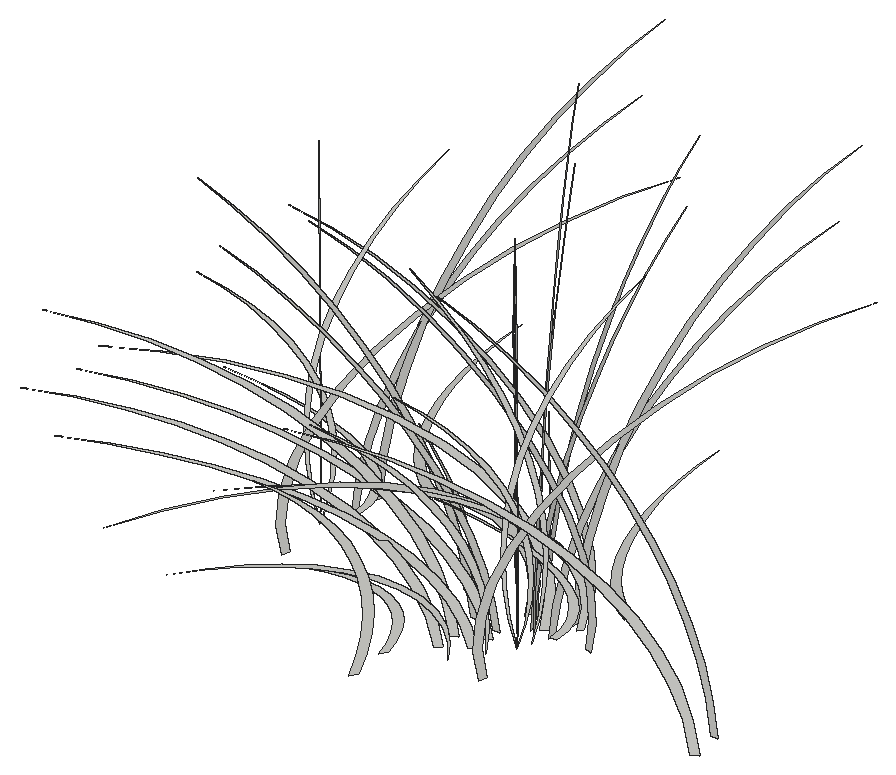
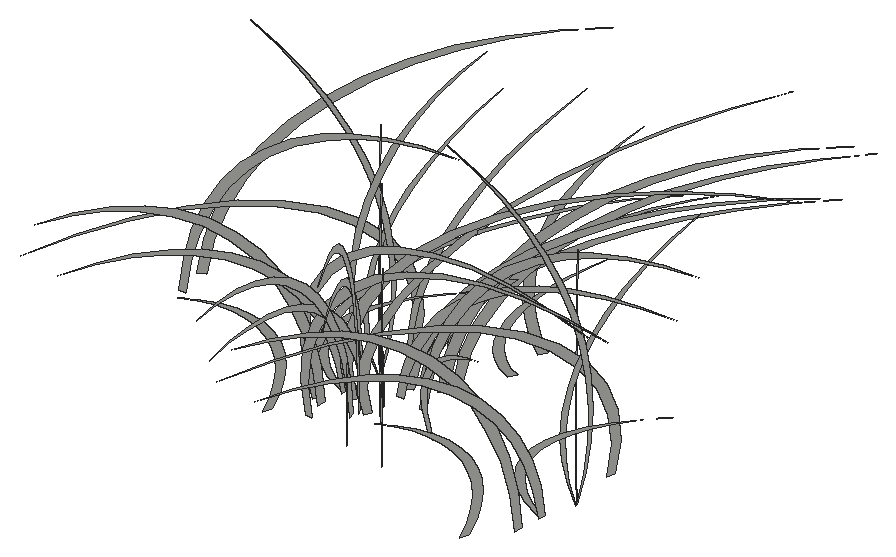
# SketchUp Ruby script. Lengths in inches.
U = 1.inch
M = Sketchup.active_model
def pt(a) = Geom::Point3d.new(a.map { |v| v * U })
def face(e, loops, mat)
  f = e.add_face(loops[0].map { |a| pt(a) })
  loops[1..].each { |l| e.add_face(l.map { |a| pt(a) }).erase! }
  f.material = f.back_material = mat if mat
  f
end
# faces: each face lists its corners as indices into pts; further lists are holes
def faces(e, pts, list, mat = nil) = list.each { |f| face(e, (f[0].is_a?(Array) ? f : [f]).map { |l| l.map { |i| pts[i] } }, mat) }
# xy, xz, yz: faces in a plane at the given z, y or x. An outline is a flat list of corners, or four numbers for a rectangle; further outlines are holes
def ring(l) = l.size == 4 ? [[l[0], l[1]], [l[2], l[1]], [l[2], l[3]], [l[0], l[3]]] : l.each_slice(2).to_a
def flat(e, list, mat, &to3) = list.each { |f| face(e, (f[0].is_a?(Array) ? f : [f]).map { |l| ring(l).map { |u, v| to3.(u, v) } }, mat) }
def xy(e, z, list, mat = nil) = flat(e, list, mat) { |x, y| [x, y, z] }
def xz(e, y, list, mat = nil) = flat(e, list, mat) { |x, z| [x, y, z] }
def yz(e, x, list, mat = nil) = flat(e, list, mat) { |y, z| [x, y, z] }
def lines(e, pts, list) = list.each { |a, b| e.add_line(pt(pts[a]), pt(pts[b])) }
# prism: a flat outline (further loops are holes) pulled along v
def prism(e, loops, v, mat = nil)
  f = face(e, loops, mat); d = Geom::Vector3d.new(v.map { |x| x * U })
  f.pushpull(f.normal.samedirection?(d) ? d.length : -d.length)
end
def box(e, o, s, mat = nil) = prism(e, [[o, [o[0] + s[0], o[1], o[2]], [o[0] + s[0], o[1] + s[1], o[2]], [o[0], o[1] + s[1], o[2]]]], [0, 0, s[2]], mat)
def at(x, y, z, deg = 0) = Geom::Transformation.translation(pt([x, y, z])) * Geom::Transformation.rotation(ORIGIN, Z_AXIS, deg.degrees)
def axes(o, x, y, z) = Geom::Transformation.new([*x, 0, *y, 0, *z, 0, *pt(o).to_a, 1])
def part(name) = M.definitions.add(name)
# library, detail: a bought-in or finely detailed component or shape, given as its bounding box
def library(name, o, s) = part(name).tap { |d| box(d.entities, o, s) }
def detail(e, o, s) = box(e.add_group.entities, o, s)
def put(e, d, t, mat = nil) = e.add_instance(d, t).tap { |i| i.material = mat if mat }
def group(e, t, mat = nil) = e.add_group.tap { |g| g.transformation = t; g.material = mat if mat }.entities
root = M.entities
g1 = group(root,at(405.82,272.46,0))
p = [[-9.01,-2.98,7.88],[-7.3,-2.41,7.38],[-5.75,-1.9,6.83],[-4.38,-1.45,6.24],[-3.2,-1.06,5.62],[-2.23,-0.74,4.96],
  [-1.47,-0.49,4.27],[-0.92,-0.31,3.57],[-0.61,-0.2,2.86],[-0.51,-0.17,2.13],[-0.65,-0.21,1.41],[-1.01,-0.33,0.7],
  [-1.6,-0.53,0],[-1.21,-0.4,0],[-0.54,-0.18,0.69],[-0.12,-0.04,1.4],[0.06,0.02,2.13],[-0.02,-0.01,2.85],
  [-0.35,-0.11,3.58],[-0.92,-0.3,4.29],[-1.73,-0.57,4.98],[-2.78,-0.92,5.64],[-4.05,-1.34,6.27],[-5.52,-1.82,6.86],
  [-7.18,-2.375,7.4]]
faces(g1,p,[[0,1,2,3,4,5,6,7,8,9,10,11,12,13,14,15,16,17,18,19,20,21,22,23,24]])
g2 = group(root,at(404.15,269.07,0))
p = [[-0.6,0.73,0],[-0.27,0.33,1.77],[-0.07,0.08,3.57],[0,0,5.36],[-0.07,0.08,7.16],[-0.27,0.32,8.95],
  [-0.6,0.73,10.73],[-1.06,1.29,12.48],[-1.65,2.01,14.2],[-2.37,2.88,15.88],[-3.21,3.91,17.52],[-4.17,5.08,19.1],
  [-5.25,6.39,20.625],[-4.23,5.15,19.08],[-3.33,4.05,17.48],[-2.53,3.08,15.83],[-1.84,2.25,14.15],[-1.27,1.55,12.43],
  [-0.82,1,10.6875],[-0.48,0.59,8.92],[-0.27,0.32,7.14],[-0.17,0.21,5.35],[-0.19,0.24,3.5625],[-0.34,0.41,1.78]]
faces(g2,p,[[0,1,2,3,4,5,6,7,8,9,10,11,12,13,14,15,16,17,18,19,20,21,22,23]])
g3 = group(root,at(404.07,270.6,0))
p = [[-0.52,-0.79,0],[-0.23,-0.35,1.51],[-0.06,-0.09,3.03],[0,0,4.56],[-0.06,-0.09,6.09],[-0.23,-0.35,7.61],
  [-0.52,-0.79,9.12],[-0.92,-1.39,10.61],[-1.43,-2.17,12.07],[-2.05,-3.12,13.5],[-2.78,-4.23,14.89],[-3.61,-5.49,16.24],
  [-4.54,-6.91,17.53],[-3.66,-5.57,16.21],[-2.88,-4.38,14.86],[-2.1875,-3.33,13.46],[-1.6,-2.43,12.03],[-1.1,-1.68,10.57],
  [-0.71,-1.08,9.08],[-0.42,-0.64,7.58],[-0.23,-0.35,6.07],[-0.15,-0.22,4.55],[-0.17,-0.25,3.03],[-0.29,-0.44,1.51]]
faces(g3,p,[[0,1,2,3,4,5,6,7,8,9,10,11,12,13,14,15,16,17,18,19,20,21,22,23]])
g4 = group(root,at(404.18,271.82,0))
p = [[1.63,20.71,16.73],[1.875,23.84,17.17],[1.64,20.8125,16.64],[1.41,17.89,15.9],[1.1875,15.1,14.96],[0.98,12.48,13.84],
  [0.79,10.06,12.54],[0.62,7.86,11.08],[0.47,5.91,9.48],[0.33,4.23,7.76],[0.22,2.84,5.92],[0.14,1.75,4.01],
  [0.08,0.98,2.02],[0.04,0.54,0],[0,0,0],[0.03,0.36,2.07],[0.09,1.09,4.1],[0.17,2.15,6.07],
  [0.28,3.55,7.94],[0.41,5.27,9.7],[0.57,7.28,11.33],[0.75,9.55,12.79],[0.95,12.07,14.08],[1.16,14.79,15.17],
  [1.39,17.68,16.0625]]
faces(g4,p,[[0,1,2,3,4,5,6,7,8,9,10,11,12,13,14,15,16,17,18,19,20,21,22,23,24]])
g5 = group(root,at(404.33,273.75,0))
p = [[1.63,20.71,20.75],[1.875,23.84,21.3],[1.64,20.8125,20.63],[1.41,17.89,19.72],[1.1875,15.1,18.55],[0.98,12.48,17.16],
  [0.79,10.06,15.55],[0.62,7.86,13.74],[0.47,5.91,11.76],[0.33,4.23,9.62],[0.22,2.84,7.35],[0.14,1.75,4.97],
  [0.08,0.98,2.51],[0.04,0.54,0],[0,0,0],[0.03,0.36,2.57],[0.09,1.09,5.09],[0.17,2.15,7.53],
  [0.28,3.55,9.85],[0.41,5.27,12.03],[0.57,7.28,14.04],[0.75,9.55,15.86],[0.95,12.07,17.46],[1.16,14.79,18.82],
  [1.39,17.68,19.92]]
faces(g5,p,[[0,1,2,3,4,5,6,7,8,9,10,11,12,13,14,15,16,17,18,19,20,21,22,23,24]])
g6 = group(root,at(417.41,266.61,0))
p = [[-20.46,3.64,18.05],[-23.54,4.19,18.53],[-20.55,3.66,17.95],[-17.67,3.15,17.15],[-14.91,2.66,16.14],[-12.33,2.2,14.93],
  [-9.93,1.77,13.53],[-7.76,1.38,11.96],[-5.84,1.04,10.23],[-4.18,0.74,8.37],[-2.8,0.5,6.39],[-1.73,0.31,4.32],
  [-0.97,0.17,2.18],[-0.53,0.09,0],[0,0,0],[-0.36,0.0625,2.23],[-1.07,0.19,4.43],[-2.125,0.38,6.55],
  [-3.51,0.625,8.57],[-5.2,0.93,10.47],[-7.1875,1.28,12.22],[-9.43,1.68,13.8],[-11.92,2.125,15.1875],[-14.61,2.6,16.37],
  [-17.46,3.11,17.33]]
faces(g6,p,[[0,1,2,3,4,5,6,7,8,9,10,11,12,13,14,15,16,17,18,19,20,21,22,23,24]])
g7 = group(root,at(402.88,269.13,0))
p = [[0.67,0.67,0],[0.3,0.3,2.04],[0.08,0.08,4.1],[0,0,6.17],[0.07,0.07,8.23],[0.3,0.3,10.29],
  [0.66,0.66,12.33],[1.18,1.18,14.34],[1.84,1.84,16.32],[2.64,2.64,18.26],[3.58,3.58,20.14],[4.65,4.65,21.96],
  [5.84,5.84,23.71],[4.72,4.72,21.93],[3.71,3.71,20.09],[2.82,2.82,18.2],[2.05,2.05,16.26],[1.42,1.42,14.29],
  [0.91,0.91,12.29],[0.54,0.54,10.26],[0.3,0.3,8.21],[0.1875,0.1875,6.15],[0.22,0.22,4.09],[0.375,0.375,2.04]]
faces(g7,p,[[0,1,2,3,4,5,6,7,8,9,10,11,12,13,14,15,16,17,18,19,20,21,22,23]])
g8 = group(root,at(405.87,275.35,0))
p = [[2.34,6.79,9.0625],[1.91,5.55,8.49],[1.52,4.43,7.85],[1.18,3.44,7.18],[0.89,2.58,6.45],[0.65,1.88,5.7],
  [0.46,1.33,4.91],[0.32,0.93,4.1],[0.24,0.7,3.28],[0.22,0.64,2.45],[0.25,0.74,1.625],[0.34,1,0.8],
  [0.49,1.42,0],[0.3,0.875,0],[0.14,0.4,0.81],[0.04,0.11,1.65],[0,0,2.49],[0.03,0.07,3.34],
  [0.11,0.33,4.17],[0.27,0.77,4.99],[0.48,1.38,5.79],[0.75,2.17,6.54],[1.07,3.11,7.26],[1.45,4.2,7.92],
  [1.87,5.43,8.52]]
faces(g8,p,[[0,1,2,3,4,5,6,7,8,9,10,11,12,13,14,15,16,17,18,19,20,21,22,23,24]])
g9 = group(root,at(417.8,264.51,0))
p = [[-18.45,-9.5625,18.05],[-21.23,-11,18.53],[-18.53,-9.61,17.95],[-15.93,-8.26,17.15],[-13.45,-6.97,16.14],[-11.12,-5.76,14.93],
  [-8.96,-4.64,13.53],[-7,-3.63,11.96],[-5.26,-2.73,10.23],[-3.77,-1.95,8.37],[-2.53,-1.3125,6.39],[-1.5625,-0.81,4.32],
  [-0.875,-0.45,2.18],[-0.48,-0.25,0],[0,0,0],[-0.32,-0.17,2.23],[-0.97,-0.5,4.43],[-1.92,-0.99,6.55],
  [-3.16,-1.64,8.57],[-4.69,-2.43,10.47],[-6.48,-3.36,12.22],[-8.51,-4.41,13.8],[-10.75,-5.57,15.1875],[-13.17,-6.83,16.37],
  [-15.75,-8.16,17.33]]
faces(g9,p,[[0,1,2,3,4,5,6,7,8,9,10,11,12,13,14,15,16,17,18,19,20,21,22,23,24]])
g10 = group(root,at(417.8,264.51,0))
p = [[-18.45,-9.5625,18.05],[-21.23,-11,18.53],[-18.53,-9.61,17.95],[-15.93,-8.26,17.15],[-13.45,-6.97,16.14],[-11.12,-5.76,14.93],
  [-8.96,-4.64,13.53],[-7,-3.63,11.96],[-5.26,-2.73,10.23],[-3.77,-1.95,8.37],[-2.53,-1.3125,6.39],[-1.5625,-0.81,4.32],
  [-0.875,-0.45,2.18],[-0.48,-0.25,0],[0,0,0],[-0.32,-0.17,2.23],[-0.97,-0.5,4.43],[-1.92,-0.99,6.55],
  [-3.16,-1.64,8.57],[-4.69,-2.43,10.47],[-6.48,-3.36,12.22],[-8.51,-4.41,13.8],[-10.75,-5.57,15.1875],[-13.17,-6.83,16.37],
  [-15.75,-8.16,17.33]]
faces(g10,p,[[0,1,2,3,4,5,6,7,8,9,10,11,12,13,14,15,16,17,18,19,20,21,22,23,24]])
g11 = group(root,at(419.3125,266.27,0))
p = [[-20.46,3.64,14.56],[-23.54,4.19,14.94],[-20.55,3.66,14.48],[-17.67,3.15,13.83],[-14.91,2.66,13.02],[-12.33,2.2,12.04],
  [-9.93,1.77,10.91],[-7.76,1.38,9.64],[-5.84,1.04,8.25],[-4.18,0.74,6.75],[-2.8,0.5,5.15],[-1.73,0.31,3.49],
  [-0.97,0.17,1.76],[-0.53,0.09,0],[0,0,0],[-0.36,0.0625,1.8],[-1.07,0.19,3.57],[-2.125,0.38,5.28],
  [-3.51,0.625,6.91],[-5.2,0.93,8.44],[-7.1875,1.28,9.85],[-9.43,1.68,11.13],[-11.92,2.125,12.25],[-14.61,2.6,13.2],
  [-17.46,3.11,13.97]]
faces(g11,p,[[0,1,2,3,4,5,6,7,8,9,10,11,12,13,14,15,16,17,18,19,20,21,22,23,24]])
g12 = group(root,at(404.03,265.19,0))
p = [[0.26,0.96,0],[0.11,0.43,0],[0,0,2.01],[0.05,0.17,4.04],[0.25,0.9375,6.02],[0.62,2.28,7.92],
  [1.125,4.16,9.68],[1.76,6.54,11.26],[2.52,9.35,12.62],[3.38,12.53,13.73],[4.32,16,14.5625],[5.31,19.67,15.09],
  [6.33,23.45,15.31],[7.35,27.24,15.2],[6.35,23.52,15.22],[5.35,19.83,14.94],[4.39,16.27,14.37],[3.48,12.91,13.51],
  [2.65,9.83,12.39],[1.92,7.11,11.04],[1.29,4.8,9.48],[0.8,2.96,7.75],[0.44,1.63,5.9],[0.23,0.84,3.96],
  [0.17,0.62,1.98]]
faces(g12,p,[[0,1,2,3,4,5,6,7,8,9,10,11,12,13,14,15,16,17,18,19,20,21,22,23,24]])
g13 = group(root,at(417.84,263.02,0))
p = [[-17.17,-11.7,15.34],[-19.76,-13.47,15.75],[-17.25,-11.76,15.26],[-14.83,-10.11,14.58],[-12.52,-8.53,13.72],[-10.35,-7.05,12.69],
  [-8.34,-5.68,11.5],[-6.52,-4.44,10.16],[-4.9,-3.34,8.7],[-3.51,-2.39,7.11],[-2.35,-1.6,5.43],[-1.45,-0.99,3.67],
  [-0.82,-0.56,1.86],[-0.45,-0.3,0],[0,0,0],[-0.3,-0.21,1.9],[-0.9,-0.61,3.76],[-1.78,-1.22,5.57],
  [-2.95,-2.01,7.28],[-4.37,-2.98,8.9],[-6.03,-4.11,10.39],[-7.92,-5.4,11.73],[-10,-6.82,12.91],[-12.26,-8.36,13.91],
  [-14.66,-9.99,14.73]]
faces(g13,p,[[0,1,2,3,4,5,6,7,8,9,10,11,12,13,14,15,16,17,18,19,20,21,22,23,24]])
g14 = group(root,at(419.52,265.4,0))
p = [[-18.45,-9.5625,14.56],[-21.23,-11,14.94],[-18.53,-9.61,14.48],[-15.93,-8.26,13.83],[-13.45,-6.97,13.02],[-11.12,-5.76,12.04],
  [-8.96,-4.64,10.91],[-7,-3.63,9.64],[-5.26,-2.73,8.25],[-3.77,-1.95,6.75],[-2.53,-1.3125,5.15],[-1.5625,-0.81,3.49],
  [-0.875,-0.45,1.76],[-0.48,-0.25,0],[0,0,0],[-0.32,-0.17,1.8],[-0.97,-0.5,3.57],[-1.92,-0.99,5.28],
  [-3.16,-1.64,6.91],[-4.69,-2.43,8.44],[-6.48,-3.36,9.85],[-8.51,-4.41,11.13],[-10.75,-5.57,12.25],[-13.17,-6.83,13.2],
  [-15.75,-8.16,13.97]]
faces(g14,p,[[0,1,2,3,4,5,6,7,8,9,10,11,12,13,14,15,16,17,18,19,20,21,22,23,24]])
g15 = group(root,at(419.52,265.4,0))
p = [[-18.45,-9.5625,14.56],[-21.23,-11,14.94],[-18.53,-9.61,14.48],[-15.93,-8.26,13.83],[-13.45,-6.97,13.02],[-11.12,-5.76,12.04],
  [-8.96,-4.64,10.91],[-7,-3.63,9.64],[-5.26,-2.73,8.25],[-3.77,-1.95,6.75],[-2.53,-1.3125,5.15],[-1.5625,-0.81,3.49],
  [-0.875,-0.45,1.76],[-0.48,-0.25,0],[0,0,0],[-0.32,-0.17,1.8],[-0.97,-0.5,3.57],[-1.92,-0.99,5.28],
  [-3.16,-1.64,6.91],[-4.69,-2.43,8.44],[-6.48,-3.36,9.85],[-8.51,-4.41,11.13],[-10.75,-5.57,12.25],[-13.17,-6.83,13.2],
  [-15.75,-8.16,13.97]]
faces(g15,p,[[0,1,2,3,4,5,6,7,8,9,10,11,12,13,14,15,16,17,18,19,20,21,22,23,24]])
g16 = group(root,at(422.38,271.12,0))
p = [[-0.91,0.16,0],[-0.4,0.07,0],[0,0,2.0625],[-0.16,0.03,4.13],[-0.89,0.16,6.16],[-2.17,0.39,8.1],
  [-3.95,0.7,9.91],[-6.21,1.11,11.52],[-8.88,1.58,12.92],[-11.91,2.12,14.05],[-15.2,2.71,14.9],[-18.68,3.33,15.45],
  [-22.27,3.97,15.67],[-25.88,4.61,15.5625],[-22.34,3.98,15.58],[-18.84,3.36,15.29],[-15.45,2.75,14.71],[-12.26,2.18,13.83],
  [-9.34,1.66,12.68],[-6.75,1.2,11.3],[-4.56,0.8125,9.7],[-2.81,0.5,7.9375],[-1.55,0.28,6.04],[-0.8,0.14,4.05],
  [-0.59,0.1,2.02]]
faces(g16,p,[[0,1,2,3,4,5,6,7,8,9,10,11,12,13,14,15,16,17,18,19,20,21,22,23,24]])
g17 = group(root,at(422.38,271.12,0))
p = [[-0.91,0.16,0],[-0.4,0.07,0],[0,0,2.0625],[-0.16,0.03,4.13],[-0.89,0.16,6.16],[-2.17,0.39,8.1],
  [-3.95,0.7,9.91],[-6.21,1.11,11.52],[-8.88,1.58,12.92],[-11.91,2.12,14.05],[-15.2,2.71,14.9],[-18.68,3.33,15.45],
  [-22.27,3.97,15.67],[-25.88,4.61,15.5625],[-22.34,3.98,15.58],[-18.84,3.36,15.29],[-15.45,2.75,14.71],[-12.26,2.18,13.83],
  [-9.34,1.66,12.68],[-6.75,1.2,11.3],[-4.56,0.8125,9.7],[-2.81,0.5,7.9375],[-1.55,0.28,6.04],[-0.8,0.14,4.05],
  [-0.59,0.1,2.02]]
faces(g17,p,[[0,1,2,3,4,5,6,7,8,9,10,11,12,13,14,15,16,17,18,19,20,21,22,23,24]])
g18 = group(root,at(419.44,264.11,0))
p = [[-17.17,-11.7,12.375],[-19.76,-13.47,12.7],[-17.25,-11.76,12.31],[-14.83,-10.11,11.76],[-12.52,-8.53,11.07],[-10.35,-7.05,10.23],
  [-8.34,-5.68,9.27],[-6.52,-4.44,8.2],[-4.9,-3.34,7.01],[-3.51,-2.39,5.74],[-2.35,-1.6,4.38],[-1.45,-0.99,2.96],
  [-0.82,-0.56,1.5],[-0.45,-0.3,0],[0,0,0],[-0.3,-0.21,1.53],[-0.9,-0.61,3.03],[-1.78,-1.22,4.49],
  [-2.95,-2.01,5.875],[-4.37,-2.98,7.18],[-6.03,-4.11,8.375],[-7.92,-5.4,9.46],[-10,-6.82,10.41],[-12.26,-8.36,11.22],
  [-14.66,-9.99,11.88]]
faces(g18,p,[[0,1,2,3,4,5,6,7,8,9,10,11,12,13,14,15,16,17,18,19,20,21,22,23,24]])
g19 = group(root,at(421.64,268.42,0))
p = [[-0.82,-0.43,0],[-0.36,-0.1875,0],[0,0,2.0625],[-0.15,-0.08,4.13],[-0.8,-0.42,6.16],[-1.95,-1.01,8.1],
  [-3.57,-1.85,9.91],[-5.6,-2.9,11.52],[-8.01,-4.15,12.92],[-10.74,-5.57,14.05],[-13.71,-7.1,14.9],[-16.85,-8.73,15.45],
  [-20.09,-10.41,15.67],[-23.34,-12.1,15.5625],[-20.15,-10.44,15.58],[-16.99,-8.81,15.29],[-13.9375,-7.22,14.71],[-11.06,-5.73,13.83],
  [-8.42,-4.37,12.68],[-6.09,-3.16,11.3],[-4.11,-2.13,9.7],[-2.53,-1.3125,7.9375],[-1.4,-0.72,6.04],[-0.72,-0.375,4.05],
  [-0.53,-0.27,2.02]]
faces(g19,p,[[0,1,2,3,4,5,6,7,8,9,10,11,12,13,14,15,16,17,18,19,20,21,22,23,24]])
g20 = group(root,at(425.23,267.56,0))
p = [[-0.95,0.28,0],[-0.42,0.125,0],[0,0,2.01],[-0.17,0.05,4.04],[-0.93,0.27,6.02],[-2.27,0.66,7.92],
  [-4.14,1.21,9.68],[-6.5,1.9,11.26],[-9.3,2.72,12.62],[-12.46,3.64,13.73],[-15.91,4.65,14.5625],[-19.55,5.72,15.09],
  [-23.3125,6.82,15.31],[-27.08,7.92,15.2],[-23.38,6.84,15.22],[-19.72,5.77,14.94],[-16.17,4.73,14.37],[-12.83,3.75,13.51],
  [-9.77,2.86,12.39],[-7.0625,2.07,11.04],[-4.77,1.39,9.48],[-2.94,0.86,7.75],[-1.62,0.47,5.9],[-0.84,0.25,3.96],
  [-0.61,0.18,1.98]]
faces(g20,p,[[0,1,2,3,4,5,6,7,8,9,10,11,12,13,14,15,16,17,18,19,20,21,22,23,24]])
g21 = group(root,at(415.97,268.3,0))
p = [[-6.53,2.99,7.88],[-5.33,2.44,7.38],[-4.26,1.95,6.83],[-3.3,1.51,6.24],[-2.48,1.14,5.62],[-1.81,0.83,4.96],
  [-1.28,0.58,4.27],[-0.9,0.41,3.57],[-0.68,0.31,2.86],[-0.61,0.28,2.13],[-0.71,0.32,1.41],[-0.96,0.4375,0.7],
  [-1.37,0.625,0],[-0.84,0.38,0],[-0.39,0.18,0.71],[-0.11,0.05,1.43],[0,0,2.17],[-0.07,0.03,2.9],
  [-0.32,0.15,3.63],[-0.74,0.34,4.34],[-1.33,0.61,5.03],[-2.08,0.95,5.69],[-2.99,1.37,6.3125],[-4.04,1.85,6.89],
  [-5.22,2.39,7.41]]
faces(g21,p,[[0,1,2,3,4,5,6,7,8,9,10,11,12,13,14,15,16,17,18,19,20,21,22,23,24]])
g22 = group(root,at(418.73,268.53,0))
p = [[-10.66,12.98,9.9],[-9.23,11.23,9.83],[-7.82,9.52,9.59],[-6.46,7.86,9.18],[-5.18,6.3,8.61],[-3.99,4.86,7.88],
  [-2.93,3.57,7.02],[-2.02,2.46,6.03],[-1.27,1.54,4.95],[-0.6875,0.84,3.78],[-0.29,0.36,2.55],[-0.1,0.12,1.28],
  [-0.09,0.12,0],[0,0,1.3],[-0.125,0.15,2.61],[-0.47,0.57,3.875],[-1.02,1.24,5.09],[-1.77,2.15,6.21],
  [-2.69,3.28,7.22],[-3.78,4.6,8.1],[-5,6.09,8.82],[-6.33,7.71,9.37],[-7.74,9.43,9.74],[-9.2,11.19,9.92]]
faces(g22,p,[[0,1,2,3,4,5,6,7,8,9,10,11,12,13,14,15,16,17,18,19,20,21,22,23]])
g23 = group(root,at(419.98,268.8,0))
p = [[-11.32,17.43,20.75],[-13.02,20.05,21.3],[-11.37,17.51,20.63],[-9.77,15.05,19.72],[-8.25,12.7,18.55],[-6.82,10.5,17.16],
  [-5.5,8.46,15.55],[-4.29,6.61,13.74],[-3.23,4.97,11.76],[-2.3125,3.56,9.62],[-1.55,2.39,7.35],[-0.96,1.47,4.97],
  [-0.54,0.83,2.51],[-0.29,0.45,0],[0,0,0],[-0.2,0.31,2.57],[-0.59,0.91,5.09],[-1.18,1.8125,7.53],
  [-1.94,2.99,9.85],[-2.88,4.43,12.03],[-3.98,6.12,14.04],[-5.22,8.04,15.86],[-6.59,10.15,17.46],[-8.08,12.44,18.82],
  [-9.66,14.88,19.92]]
faces(g23,p,[[0,1,2,3,4,5,6,7,8,9,10,11,12,13,14,15,16,17,18,19,20,21,22,23,24]])
g24 = group(root,at(415.86,272.02,0))
p = [[-4.56,5.55,16.02],[-3.72,4.53,15.01],[-2.97,3.62,13.89],[-2.31,2.81,12.69],[-1.73,2.11,11.42],[-1.26,1.54,10.08],
  [-0.89,1.09,8.6875],[-0.63,0.76,7.26],[-0.47,0.58,5.8],[-0.43,0.52,4.34],[-0.49,0.6,2.87],[-0.67,0.81,1.42],
  [-0.95,1.16,0],[-0.59,0.71,0],[-0.27,0.33,1.44],[-0.07,0.09,2.92],[0,0,4.41],[-0.05,0.0625,5.9],
  [-0.22,0.27,7.38],[-0.52,0.63,8.83],[-0.93,1.13,10.23],[-1.45,1.77,11.57],[-2.09,2.54,12.83],[-2.82,3.43,14.01],
  [-3.65,4.44,15.07]]
faces(g24,p,[[0,1,2,3,4,5,6,7,8,9,10,11,12,13,14,15,16,17,18,19,20,21,22,23,24]])
g25 = group(root,at(415.86,272.02,0))
p = [[-4.56,5.55,16.02],[-3.72,4.53,15.01],[-2.97,3.62,13.89],[-2.31,2.81,12.69],[-1.73,2.11,11.42],[-1.26,1.54,10.08],
  [-0.89,1.09,8.6875],[-0.63,0.76,7.26],[-0.47,0.58,5.8],[-0.43,0.52,4.34],[-0.49,0.6,2.87],[-0.67,0.81,1.42],
  [-0.95,1.16,0],[-0.59,0.71,0],[-0.27,0.33,1.44],[-0.07,0.09,2.92],[0,0,4.41],[-0.05,0.0625,5.9],
  [-0.22,0.27,7.38],[-0.52,0.63,8.83],[-0.93,1.13,10.23],[-1.45,1.77,11.57],[-2.09,2.54,12.83],[-2.82,3.43,14.01],
  [-3.65,4.44,15.07]]
faces(g25,p,[[0,1,2,3,4,5,6,7,8,9,10,11,12,13,14,15,16,17,18,19,20,21,22,23,24]])
g26 = group(root,at(419.55,269.61,0))
p = [[-0.37,-0.92,0],[-0.16,-0.41,0],[0,0,1.75],[-0.07,-0.17,3.51],[-0.36,-0.9,5.24],[-0.88,-2.19,6.89],
  [-1.61,-4,8.42],[-2.53,-6.28,9.8],[-3.61,-8.99,10.98],[-4.84,-12.04,11.95],[-6.18,-15.375,12.67],[-7.6,-18.9,13.13],
  [-9.06,-22.53,13.32],[-10.53,-26.18,13.23],[-9.09,-22.6,13.25],[-7.66,-19.06,13],[-6.29,-15.63,12.5],[-4.99,-12.41,11.75],
  [-3.8,-9.45,10.78],[-2.75,-6.83,9.6],[-1.85,-4.61,8.25],[-1.14,-2.84,6.75],[-0.63,-1.57,5.13],[-0.33,-0.8125,3.44],
  [-0.24,-0.59,1.72]]
faces(g26,p,[[0,1,2,3,4,5,6,7,8,9,10,11,12,13,14,15,16,17,18,19,20,21,22,23,24]])
g27 = group(root,at(416.3,261.43,0))
p = [[-3.94,-6,6.7],[-3.22,-4.9,6.27],[-2.57,-3.91,5.81],[-2,-3.04,5.31],[-1.5,-2.28,4.77],[-1.09,-1.66,4.21],
  [-0.77,-1.17,3.63],[-0.54,-0.83,3.03],[-0.41,-0.62,2.43],[-0.37,-0.5625,1.8125],[-0.43,-0.65,1.2],[-0.58,-0.88,0.59],
  [-0.83,-1.26,0],[-0.51,-0.77,0],[-0.23,-0.36,0.6],[-0.0625,-0.1,1.22],[0,0,1.84],[-0.04,-0.07,2.47],
  [-0.19,-0.29,3.09],[-0.45,-0.68,3.69],[-0.8,-1.22,4.28],[-1.26,-1.91,4.84],[-1.81,-2.75,5.37],[-2.44,-3.71,5.86],
  [-3.16,-4.8,6.3]]
faces(g27,p,[[0,1,2,3,4,5,6,7,8,9,10,11,12,13,14,15,16,17,18,19,20,21,22,23,24]])
g28 = group(root,at(419.07,262.12,0))
p = [[-9.23,-14.04,8.41],[-7.99,-12.15,8.36],[-6.77,-10.29,8.15],[-5.59,-8.5,7.8],[-4.48,-6.8125,7.32],[-3.46,-5.26,6.7],
  [-2.54,-3.86,5.97],[-1.75,-2.66,5.13],[-1.09,-1.67,4.2],[-0.59,-0.9,3.21],[-0.25,-0.39,2.16],[-0.08,-0.125,1.09],
  [-0.08,-0.125,0],[0,0,1.11],[-0.11,-0.16,2.21],[-0.4,-0.61,3.29],[-0.88,-1.34,4.32],[-1.53,-2.33,5.28],
  [-2.33,-3.55,6.14],[-3.27,-4.98,6.88],[-4.33,-6.59,7.5],[-5.48,-8.34,7.97],[-6.7,-10.19,8.28],[-7.96,-12.11,8.43]]
faces(g28,p,[[0,1,2,3,4,5,6,7,8,9,10,11,12,13,14,15,16,17,18,19,20,21,22,23]])
g29 = group(root,at(421.04,267.18,0))
p = [[-11.32,17.43,16.73],[-13.02,20.05,17.17],[-11.37,17.51,16.64],[-9.77,15.05,15.9],[-8.25,12.7,14.96],[-6.82,10.5,13.84],
  [-5.5,8.46,12.54],[-4.29,6.61,11.08],[-3.23,4.97,9.48],[-2.3125,3.56,7.76],[-1.55,2.39,5.92],[-0.96,1.47,4.01],
  [-0.54,0.83,2.02],[-0.29,0.45,0],[0,0,0],[-0.2,0.31,2.07],[-0.59,0.91,4.1],[-1.18,1.8125,6.07],
  [-1.94,2.99,7.94],[-2.88,4.43,9.7],[-3.98,6.12,11.33],[-5.22,8.04,12.79],[-6.59,10.15,14.08],[-8.08,12.44,15.17],
  [-9.66,14.88,16.0625]]
faces(g29,p,[[0,1,2,3,4,5,6,7,8,9,10,11,12,13,14,15,16,17,18,19,20,21,22,23,24]])
g30 = group(root,at(416.59,258.35,0))
p = [[-3.94,-6,13.62],[-3.22,-4.9,12.76],[-2.57,-3.91,11.81],[-2,-3.04,10.79],[-1.5,-2.28,9.7],[-1.09,-1.66,8.57],
  [-0.77,-1.17,7.38],[-0.54,-0.83,6.17],[-0.41,-0.62,4.93],[-0.37,-0.5625,3.6875],[-0.43,-0.65,2.44],[-0.58,-0.88,1.21],
  [-0.83,-1.26,0],[-0.51,-0.77,0],[-0.23,-0.36,1.22],[-0.0625,-0.1,2.48],[0,0,3.75],[-0.04,-0.07,5.02],
  [-0.19,-0.29,6.28],[-0.45,-0.68,7.51],[-0.8,-1.22,8.7],[-1.26,-1.91,9.84],[-1.81,-2.75,10.91],[-2.44,-3.71,11.9],
  [-3.16,-4.8,12.8125]]
faces(g30,p,[[0,1,2,3,4,5,6,7,8,9,10,11,12,13,14,15,16,17,18,19,20,21,22,23,24]])
g31 = group(root,at(423.06,269.77,0))
p = [[-0.5,-0.57,0],[-0.22,-0.25,0],[0,0,1.46],[-0.09,-0.1,2.93],[-0.49,-0.56,4.375],[-1.19,-1.35,5.75],
  [-2.17,-2.47,7.03],[-3.41,-3.89,8.18],[-4.88,-5.56,9.17],[-6.54,-7.45,9.98],[-8.36,-9.51,10.58],[-10.27,-11.69,10.97],
  [-12.24,-13.9375,11.125],[-14.23,-16.19,11.05],[-12.28,-13.98,11.0625],[-10.36,-11.79,10.86],[-8.5,-9.67,10.44],[-6.74,-7.67,9.82],
  [-5.13,-5.84,9.01],[-3.71,-4.22,8.02],[-2.51,-2.85,6.89],[-1.54,-1.76,5.64],[-0.85,-0.97,4.29],[-0.44,-0.5,2.88],
  [-0.32,-0.37,1.4375]]
faces(g31,p,[[0,1,2,3,4,5,6,7,8,9,10,11,12,13,14,15,16,17,18,19,20,21,22,23,24]])
g32 = group(root,at(423.06,269.77,0))
p = [[-0.5,-0.57,0],[-0.22,-0.25,0],[0,0,1.46],[-0.09,-0.1,2.93],[-0.49,-0.56,4.375],[-1.19,-1.35,5.75],
  [-2.17,-2.47,7.03],[-3.41,-3.89,8.18],[-4.88,-5.56,9.17],[-6.54,-7.45,9.98],[-8.36,-9.51,10.58],[-10.27,-11.69,10.97],
  [-12.24,-13.9375,11.125],[-14.23,-16.19,11.05],[-12.28,-13.98,11.0625],[-10.36,-11.79,10.86],[-8.5,-9.67,10.44],[-6.74,-7.67,9.82],
  [-5.13,-5.84,9.01],[-3.71,-4.22,8.02],[-2.51,-2.85,6.89],[-1.54,-1.76,5.64],[-0.85,-0.97,4.29],[-0.44,-0.5,2.88],
  [-0.32,-0.37,1.4375]]
faces(g32,p,[[0,1,2,3,4,5,6,7,8,9,10,11,12,13,14,15,16,17,18,19,20,21,22,23,24]])
g33 = group(root,at(419.95,269.4375,0))
p = [[-6.07,19.87,18.05],[-6.99,22.87,18.53],[-6.1,19.96,17.95],[-5.25,17.16,17.15],[-4.43,14.49,16.14],[-3.66,11.97,14.93],
  [-2.95,9.65,13.53],[-2.31,7.54,11.96],[-1.73,5.67,10.23],[-1.24,4.06,8.37],[-0.83,2.72,6.39],[-0.51,1.68,4.32],
  [-0.29,0.94,2.18],[-0.16,0.52,0],[0,0,0],[-0.11,0.35,2.23],[-0.32,1.04,4.43],[-0.63,2.07,6.55],
  [-1.04,3.41,8.57],[-1.55,5.05,10.47],[-2.13,6.98,12.22],[-2.8,9.16,13.8],[-3.54,11.58,15.1875],[-4.34,14.1875,16.37],
  [-5.1875,16.96,17.33]]
faces(g33,p,[[0,1,2,3,4,5,6,7,8,9,10,11,12,13,14,15,16,17,18,19,20,21,22,23,24]])
g34 = group(root,at(418.89,271.38,0))
p = [[-4.56,5.55,7.88],[-3.72,4.53,7.38],[-2.97,3.62,6.83],[-2.31,2.81,6.24],[-1.73,2.11,5.62],[-1.26,1.54,4.96],
  [-0.89,1.09,4.27],[-0.63,0.76,3.57],[-0.47,0.58,2.86],[-0.43,0.52,2.13],[-0.49,0.6,1.41],[-0.67,0.81,0.7],
  [-0.95,1.16,0],[-0.59,0.71,0],[-0.27,0.33,0.71],[-0.07,0.09,1.43],[0,0,2.17],[-0.05,0.0625,2.9],
  [-0.22,0.27,3.63],[-0.52,0.63,4.34],[-0.93,1.13,5.03],[-1.45,1.77,5.69],[-2.09,2.54,6.3125],[-2.82,3.43,6.89],
  [-3.65,4.44,7.41]]
faces(g34,p,[[0,1,2,3,4,5,6,7,8,9,10,11,12,13,14,15,16,17,18,19,20,21,22,23,24]])
g35 = group(root,at(420.17,266.78,0))
p = [[-6.74,8.21,19.61],[-5.67,6.9,18.16],[-4.68,5.7,16.67],[-3.78,4.6,15.125],[-2.98,3.62,13.55],[-2.27,2.76,11.93],
  [-1.65,2.01,10.28],[-1.14,1.39,8.61],[-0.72,0.88,6.91],[-0.41,0.5,5.2],[-0.2,0.24,3.47],[-0.09,0.11,1.74],
  [-0.09,0.11,0],[0,0,1.74],[-0.03,0.04,3.49],[-0.1875,0.23,5.23],[-0.46,0.56,6.96],[-0.85,1.04,8.67],
  [-1.36,1.66,10.36],[-1.98,2.42,12.01],[-2.72,3.3125,13.63],[-3.57,4.35,15.21],[-4.52,5.51,16.73],[-5.58,6.8,18.2]]
faces(g35,p,[[0,1,2,3,4,5,6,7,8,9,10,11,12,13,14,15,16,17,18,19,20,21,22,23]])
g36 = group(root,at(420.17,266.78,0))
p = [[-6.74,8.21,19.61],[-5.67,6.9,18.16],[-4.68,5.7,16.67],[-3.78,4.6,15.125],[-2.98,3.62,13.55],[-2.27,2.76,11.93],
  [-1.65,2.01,10.28],[-1.14,1.39,8.61],[-0.72,0.88,6.91],[-0.41,0.5,5.2],[-0.2,0.24,3.47],[-0.09,0.11,1.74],
  [-0.09,0.11,0],[0,0,1.74],[-0.03,0.04,3.49],[-0.1875,0.23,5.23],[-0.46,0.56,6.96],[-0.85,1.04,8.67],
  [-1.36,1.66,10.36],[-1.98,2.42,12.01],[-2.72,3.3125,13.63],[-3.57,4.35,15.21],[-4.52,5.51,16.73],[-5.58,6.8,18.2]]
faces(g36,p,[[0,1,2,3,4,5,6,7,8,9,10,11,12,13,14,15,16,17,18,19,20,21,22,23]])
g37 = group(root,at(420.52,267.59,0))
p = [[-6.07,19.87,14.56],[-6.99,22.87,14.94],[-6.1,19.96,14.48],[-5.25,17.16,13.83],[-4.43,14.49,13.02],[-3.66,11.97,12.04],
  [-2.95,9.65,10.91],[-2.31,7.54,9.64],[-1.73,5.67,8.25],[-1.24,4.06,6.75],[-0.83,2.72,5.15],[-0.51,1.68,3.49],
  [-0.29,0.94,1.76],[-0.16,0.52,0],[0,0,0],[-0.11,0.35,1.8],[-0.32,1.04,3.57],[-0.63,2.07,5.28],
  [-1.04,3.41,6.91],[-1.55,5.05,8.44],[-2.13,6.98,9.85],[-2.8,9.16,11.13],[-3.54,11.58,12.25],[-4.34,14.1875,13.2],
  [-5.1875,16.96,13.97]]
faces(g37,p,[[0,1,2,3,4,5,6,7,8,9,10,11,12,13,14,15,16,17,18,19,20,21,22,23,24]])
g38 = group(root,at(420.32,264.02,0))
p = [[-5.83,-8.875,16.67],[-4.9,-7.46,15.44],[-4.05,-6.16,14.17],[-3.27,-4.98,12.86],[-2.58,-3.92,11.51],[-1.96,-2.98,10.14],
  [-1.43,-2.18,8.74],[-0.99,-1.5,7.31],[-0.63,-0.95,5.87],[-0.36,-0.54,4.42],[-0.17,-0.26,2.95],[-0.08,-0.12,1.48],
  [-0.08,-0.12,0],[0,0,1.48],[-0.03,-0.04,2.97],[-0.16,-0.24,4.45],[-0.4,-0.6,5.92],[-0.74,-1.12,7.37],
  [-1.18,-1.79,8.81],[-1.72,-2.61,10.21],[-2.36,-3.58,11.59],[-3.09,-4.7,12.93],[-3.92,-5.96,14.22],[-4.83,-7.35,15.47]]
faces(g38,p,[[0,1,2,3,4,5,6,7,8,9,10,11,12,13,14,15,16,17,18,19,20,21,22,23]])
g39 = group(root,at(422.43,266.75,0))
p = [[-0.89,-0.32,0],[-0.4,-0.14,1.97],[-0.1,-0.04,3.96],[0,0,5.95],[-0.1,-0.03,7.95],[-0.39,-0.14,9.9375],
  [-0.89,-0.3125,11.91],[-1.57,-0.56,13.85],[-2.45,-0.87,15.76],[-3.52,-1.25,17.63],[-4.77,-1.6875,19.44],[-6.19,-2.19,21.2],
  [-7.79,-2.76,22.89],[-6.29,-2.23,21.17],[-4.94,-1.75,19.4],[-3.76,-1.33,17.58],[-2.74,-0.97,15.71],[-1.89,-0.67,13.8],
  [-1.22,-0.43,11.86],[-0.72,-0.25,9.9],[-0.4,-0.14,7.93],[-0.25,-0.09,5.94],[-0.29,-0.1,3.95],[-0.5,-0.18,1.97]]
faces(g39,p,[[0,1,2,3,4,5,6,7,8,9,10,11,12,13,14,15,16,17,18,19,20,21,22,23]])
g40 = group(root,at(423.53,268.11,0))
p = [[-9.01,-2.98,7.88],[-7.3,-2.41,7.38],[-5.75,-1.9,6.83],[-4.38,-1.45,6.24],[-3.2,-1.06,5.62],[-2.23,-0.74,4.96],
  [-1.47,-0.49,4.27],[-0.92,-0.31,3.57],[-0.61,-0.2,2.86],[-0.51,-0.17,2.13],[-0.65,-0.21,1.41],[-1.01,-0.33,0.7],
  [-1.6,-0.53,0],[-1.21,-0.4,0],[-0.54,-0.18,0.69],[-0.12,-0.04,1.4],[0.06,0.02,2.13],[-0.02,-0.01,2.85],
  [-0.35,-0.11,3.58],[-0.92,-0.3,4.29],[-1.73,-0.57,4.98],[-2.78,-0.92,5.64],[-4.05,-1.34,6.27],[-5.52,-1.82,6.86],
  [-7.18,-2.375,7.4]]
faces(g40,p,[[0,1,2,3,4,5,6,7,8,9,10,11,12,13,14,15,16,17,18,19,20,21,22,23,24]])
g41 = group(root,at(421.86,264.72,0))
p = [[-0.6,0.73,0],[-0.27,0.33,1.77],[-0.07,0.08,3.57],[0,0,5.36],[-0.07,0.08,7.16],[-0.27,0.32,8.95],
  [-0.6,0.73,10.73],[-1.06,1.29,12.48],[-1.65,2.01,14.2],[-2.37,2.88,15.88],[-3.21,3.91,17.52],[-4.17,5.08,19.1],
  [-5.25,6.39,20.625],[-4.23,5.15,19.08],[-3.33,4.05,17.48],[-2.53,3.08,15.83],[-1.84,2.25,14.15],[-1.27,1.55,12.43],
  [-0.82,1,10.6875],[-0.48,0.59,8.92],[-0.27,0.32,7.14],[-0.17,0.21,5.35],[-0.19,0.24,3.5625],[-0.34,0.41,1.78]]
faces(g41,p,[[0,1,2,3,4,5,6,7,8,9,10,11,12,13,14,15,16,17,18,19,20,21,22,23]])
g42 = group(root,at(421.78,266.24,0))
p = [[-0.52,-0.79,0],[-0.23,-0.35,1.51],[-0.06,-0.09,3.03],[0,0,4.56],[-0.06,-0.09,6.09],[-0.23,-0.35,7.61],
  [-0.52,-0.79,9.12],[-0.92,-1.39,10.61],[-1.43,-2.17,12.07],[-2.05,-3.12,13.5],[-2.78,-4.23,14.89],[-3.61,-5.49,16.24],
  [-4.54,-6.91,17.53],[-3.66,-5.57,16.21],[-2.88,-4.38,14.86],[-2.1875,-3.33,13.46],[-1.6,-2.43,12.03],[-1.1,-1.68,10.57],
  [-0.71,-1.08,9.08],[-0.42,-0.64,7.58],[-0.23,-0.35,6.07],[-0.15,-0.22,4.55],[-0.17,-0.25,3.03],[-0.29,-0.44,1.51]]
faces(g42,p,[[0,1,2,3,4,5,6,7,8,9,10,11,12,13,14,15,16,17,18,19,20,21,22,23]])
g43 = group(root,at(421.89,267.47,0))
p = [[1.63,20.71,16.73],[1.875,23.84,17.17],[1.64,20.8125,16.64],[1.41,17.89,15.9],[1.1875,15.1,14.96],[0.98,12.48,13.84],
  [0.79,10.06,12.54],[0.62,7.86,11.08],[0.47,5.91,9.48],[0.33,4.23,7.76],[0.22,2.84,5.92],[0.14,1.75,4.01],
  [0.08,0.98,2.02],[0.04,0.54,0],[0,0,0],[0.03,0.36,2.07],[0.09,1.09,4.1],[0.17,2.15,6.07],
  [0.28,3.55,7.94],[0.41,5.27,9.7],[0.57,7.28,11.33],[0.75,9.55,12.79],[0.95,12.07,14.08],[1.16,14.79,15.17],
  [1.39,17.68,16.0625]]
faces(g43,p,[[0,1,2,3,4,5,6,7,8,9,10,11,12,13,14,15,16,17,18,19,20,21,22,23,24]])
g44 = group(root,at(422.04,269.4,0))
p = [[1.63,20.71,20.75],[1.875,23.84,21.3],[1.64,20.8125,20.63],[1.41,17.89,19.72],[1.1875,15.1,18.55],[0.98,12.48,17.16],
  [0.79,10.06,15.55],[0.62,7.86,13.74],[0.47,5.91,11.76],[0.33,4.23,9.62],[0.22,2.84,7.35],[0.14,1.75,4.97],
  [0.08,0.98,2.51],[0.04,0.54,0],[0,0,0],[0.03,0.36,2.57],[0.09,1.09,5.09],[0.17,2.15,7.53],
  [0.28,3.55,9.85],[0.41,5.27,12.03],[0.57,7.28,14.04],[0.75,9.55,15.86],[0.95,12.07,17.46],[1.16,14.79,18.82],
  [1.39,17.68,19.92]]
faces(g44,p,[[0,1,2,3,4,5,6,7,8,9,10,11,12,13,14,15,16,17,18,19,20,21,22,23,24]])
g45 = group(root,at(420.59,264.78,0))
p = [[0.67,0.67,0],[0.3,0.3,2.04],[0.08,0.08,4.1],[0,0,6.17],[0.07,0.07,8.23],[0.3,0.3,10.29],
  [0.66,0.66,12.33],[1.18,1.18,14.34],[1.84,1.84,16.32],[2.64,2.64,18.26],[3.58,3.58,20.14],[4.65,4.65,21.96],
  [5.84,5.84,23.71],[4.72,4.72,21.93],[3.71,3.71,20.09],[2.82,2.82,18.2],[2.05,2.05,16.26],[1.42,1.42,14.29],
  [0.91,0.91,12.29],[0.54,0.54,10.26],[0.3,0.3,8.21],[0.1875,0.1875,6.15],[0.22,0.22,4.09],[0.375,0.375,2.04]]
faces(g45,p,[[0,1,2,3,4,5,6,7,8,9,10,11,12,13,14,15,16,17,18,19,20,21,22,23]])
g46 = group(root,at(423.58,271,0))
p = [[2.34,6.79,9.0625],[1.91,5.55,8.49],[1.52,4.43,7.85],[1.18,3.44,7.18],[0.89,2.58,6.45],[0.65,1.88,5.7],
  [0.46,1.33,4.91],[0.32,0.93,4.1],[0.24,0.7,3.28],[0.22,0.64,2.45],[0.25,0.74,1.625],[0.34,1,0.8],
  [0.49,1.42,0],[0.3,0.875,0],[0.14,0.4,0.81],[0.04,0.11,1.65],[0,0,2.49],[0.03,0.07,3.34],
  [0.11,0.33,4.17],[0.27,0.77,4.99],[0.48,1.38,5.79],[0.75,2.17,6.54],[1.07,3.11,7.26],[1.45,4.2,7.92],
  [1.87,5.43,8.52]]
faces(g46,p,[[0,1,2,3,4,5,6,7,8,9,10,11,12,13,14,15,16,17,18,19,20,21,22,23,24]])
g47 = group(root,at(436.5625,264.4,0))
p = [[-20.46,3.64,18.05],[-23.54,4.19,18.53],[-20.55,3.66,17.95],[-17.67,3.15,17.15],[-14.91,2.66,16.14],[-12.33,2.2,14.93],
  [-9.93,1.77,13.53],[-7.76,1.38,11.96],[-5.84,1.04,10.23],[-4.18,0.74,8.37],[-2.8,0.5,6.39],[-1.73,0.31,4.32],
  [-0.97,0.17,2.18],[-0.53,0.09,0],[0,0,0],[-0.36,0.0625,2.23],[-1.07,0.19,4.43],[-2.125,0.38,6.55],
  [-3.51,0.625,8.57],[-5.2,0.93,10.47],[-7.1875,1.28,12.22],[-9.43,1.68,13.8],[-11.92,2.125,15.1875],[-14.61,2.6,16.37],
  [-17.46,3.11,17.33]]
faces(g47,p,[[0,1,2,3,4,5,6,7,8,9,10,11,12,13,14,15,16,17,18,19,20,21,22,23,24]])
g48 = group(root,at(421.74,260.84,0))
p = [[0.26,0.96,0],[0.11,0.43,0],[0,0,2.01],[0.05,0.17,4.04],[0.25,0.9375,6.02],[0.62,2.28,7.92],
  [1.125,4.16,9.68],[1.76,6.54,11.26],[2.52,9.35,12.62],[3.38,12.53,13.73],[4.32,16,14.5625],[5.31,19.67,15.09],
  [6.33,23.45,15.31],[7.35,27.24,15.2],[6.35,23.52,15.22],[5.35,19.83,14.94],[4.39,16.27,14.37],[3.48,12.91,13.51],
  [2.65,9.83,12.39],[1.92,7.11,11.04],[1.29,4.8,9.48],[0.8,2.96,7.75],[0.44,1.63,5.9],[0.23,0.84,3.96],
  [0.17,0.62,1.98]]
faces(g48,p,[[0,1,2,3,4,5,6,7,8,9,10,11,12,13,14,15,16,17,18,19,20,21,22,23,24]])
g49 = group(root,at(436.95,262.29,0))
p = [[-18.45,-9.5625,18.05],[-21.23,-11,18.53],[-18.53,-9.61,17.95],[-15.93,-8.26,17.15],[-13.45,-6.97,16.14],[-11.12,-5.76,14.93],
  [-8.96,-4.64,13.53],[-7,-3.63,11.96],[-5.26,-2.73,10.23],[-3.77,-1.95,8.37],[-2.53,-1.3125,6.39],[-1.5625,-0.81,4.32],
  [-0.875,-0.45,2.18],[-0.48,-0.25,0],[0,0,0],[-0.32,-0.17,2.23],[-0.97,-0.5,4.43],[-1.92,-0.99,6.55],
  [-3.16,-1.64,8.57],[-4.69,-2.43,10.47],[-6.48,-3.36,12.22],[-8.51,-4.41,13.8],[-10.75,-5.57,15.1875],[-13.17,-6.83,16.37],
  [-15.75,-8.16,17.33]]
faces(g49,p,[[0,1,2,3,4,5,6,7,8,9,10,11,12,13,14,15,16,17,18,19,20,21,22,23,24]])
